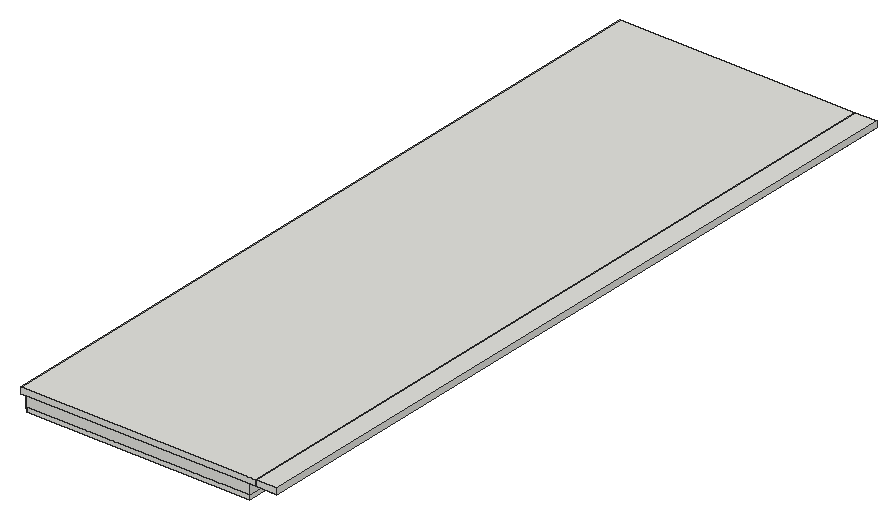
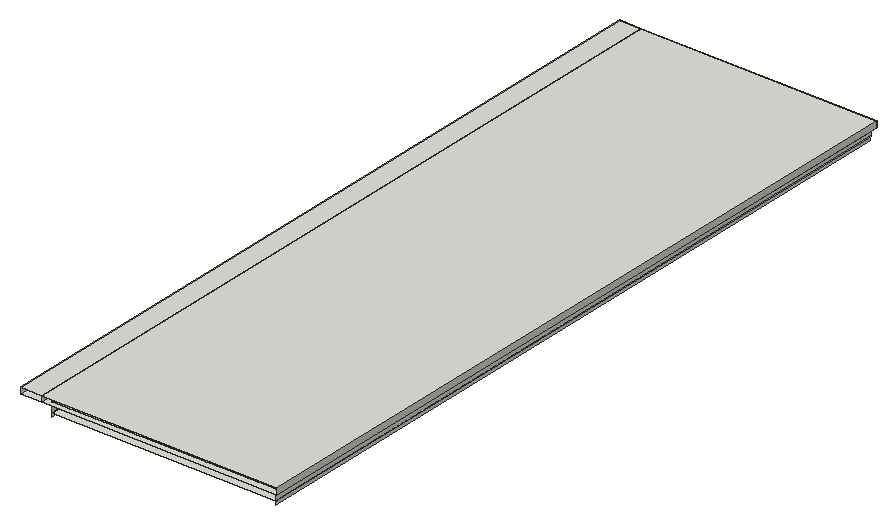
# SketchUp Ruby script. Lengths in inches.
U = 1.inch
M = Sketchup.active_model
def pt(a) = Geom::Point3d.new(a.map { |v| v * U })
def face(e, loops, mat)
  f = e.add_face(loops[0].map { |a| pt(a) })
  loops[1..].each { |l| e.add_face(l.map { |a| pt(a) }).erase! }
  f.material = f.back_material = mat if mat
  f
end
# faces: each face lists its corners as indices into pts; further lists are holes
def faces(e, pts, list, mat = nil) = list.each { |f| face(e, (f[0].is_a?(Array) ? f : [f]).map { |l| l.map { |i| pts[i] } }, mat) }
# xy, xz, yz: faces in a plane at the given z, y or x. An outline is a flat list of corners, or four numbers for a rectangle; further outlines are holes
def ring(l) = l.size == 4 ? [[l[0], l[1]], [l[2], l[1]], [l[2], l[3]], [l[0], l[3]]] : l.each_slice(2).to_a
def flat(e, list, mat, &to3) = list.each { |f| face(e, (f[0].is_a?(Array) ? f : [f]).map { |l| ring(l).map { |u, v| to3.(u, v) } }, mat) }
def xy(e, z, list, mat = nil) = flat(e, list, mat) { |x, y| [x, y, z] }
def xz(e, y, list, mat = nil) = flat(e, list, mat) { |x, z| [x, y, z] }
def yz(e, x, list, mat = nil) = flat(e, list, mat) { |y, z| [x, y, z] }
def lines(e, pts, list) = list.each { |a, b| e.add_line(pt(pts[a]), pt(pts[b])) }
# prism: a flat outline (further loops are holes) pulled along v
def prism(e, loops, v, mat = nil)
  f = face(e, loops, mat); d = Geom::Vector3d.new(v.map { |x| x * U })
  f.pushpull(f.normal.samedirection?(d) ? d.length : -d.length)
end
def box(e, o, s, mat = nil) = prism(e, [[o, [o[0] + s[0], o[1], o[2]], [o[0] + s[0], o[1] + s[1], o[2]], [o[0], o[1] + s[1], o[2]]]], [0, 0, s[2]], mat)
def at(x, y, z, deg = 0) = Geom::Transformation.translation(pt([x, y, z])) * Geom::Transformation.rotation(ORIGIN, Z_AXIS, deg.degrees)
def axes(o, x, y, z) = Geom::Transformation.new([*x, 0, *y, 0, *z, 0, *pt(o).to_a, 1])
def part(name) = M.definitions.add(name)
# library, detail: a bought-in or finely detailed component or shape, given as its bounding box
def library(name, o, s) = part(name).tap { |d| box(d.entities, o, s) }
def detail(e, o, s) = box(e.add_group.entities, o, s)
def put(e, d, t, mat = nil) = e.add_instance(d, t).tap { |i| i.material = mat if mat }
def group(e, t, mat = nil) = e.add_group.tap { |g| g.transformation = t; g.material = mat if mat }.entities
root = M.entities
xy(root,155.5,[[6,0,6.4,756.6875]])
xy(root,156.12,[[6,0,234,757.0625]])
xy(root,166.28,[[0,0,0,763.0625,240,763.0625,240,0,234,0,234,757.0625,6,757.0625,6,0],[6,0,234,757.0625],[240,0,261.625,763.0625]])
xy(root,172.28,[[0,0,240,763.0625],[240,0,261.625,763.0625]])
xz(root,0,[[6.4,152.12,234,152.12,234,156.12,6,156.12,6,155.5,6.4,155.5],[6,156.12,234,166.28],[0,166.28,240,172.28],[240,166.28,261.625,172.28]])
xz(root,551,[[57.9375,152.12,182.0625,153.65]])
yz(root,0,[[0,166.28,763.0625,172.28]])
yz(root,6,[[0,155.5,757.0625,156.12],[0,156.12,757.0625,166.28]])
yz(root,6.4,[[0,152.12,756.6875,155.5]])
yz(root,234,[[0,152.12,757.0625,156.12],[0,156.12,757.0625,166.28]])
yz(root,240,[[0,166.28,763.0625,172.28]])
yz(root,261.625,[[0,166.28,763.0625,172.28]])
p = [[59,535.0625,152.12],[57.71,535.23,152.12],[57.71,535.23,153.44],[59,535.0625,153.44],[60.29,535.23,152.12],[60.29,535.23,153.44],
  [181,535.0625,152.12],[179.71,535.23,152.12],[179.71,535.23,153.31],[181,535.0625,153.31],[182.29,535.23,152.12],[182.29,535.23,153.31],
  [56.5,535.73,152.12],[56.5,535.73,153.44],[61.5,535.73,152.12],[61.5,535.73,153.44],[178.5,535.73,152.12],[178.5,535.73,153.31],
  [183.5,535.73,152.12],[183.5,535.73,153.31],[55.46,536.53,152.12],[55.46,536.53,153.44],[62.54,536.53,152.12],[62.54,536.53,153.44],
  [177.46,536.53,152.12],[177.46,536.53,153.31],[184.54,536.53,152.12],[184.54,536.53,153.31],[54.67,537.5625,152.12],[54.67,537.5625,153.44],
  [63.33,537.5625,152.12],[63.33,537.5625,153.44],[176.67,537.5625,152.12],[176.67,537.5625,153.31],[185.33,537.5625,152.12],[185.33,537.5625,153.31],
  [54.17,538.77,152.12],[54.17,538.77,153.44],[63.83,538.77,152.12],[63.83,538.77,153.44],[176.17,538.77,152.12],[176.17,538.77,153.31],
  [185.83,538.77,152.12],[185.83,538.77,153.31],[54,540.0625,152.12],[54,540.0625,153.44],[64,540.0625,152.12],[64,540.0625,153.44],
  [176,540.0625,152.12],[176,540.0625,153.31],[186,540.0625,152.12],[186,540.0625,153.31],[54.17,541.36,152.12],[54.17,541.36,153.44],
  [63.83,541.36,152.12],[63.83,541.36,153.44],[176.17,541.36,152.12],[176.17,541.36,153.31],[185.83,541.36,152.12],[185.83,541.36,153.31],
  [54.67,542.5625,152.12],[54.67,542.5625,153.44],[63.33,542.5625,152.12],[63.33,542.5625,153.44],[176.67,542.5625,152.12],[176.67,542.5625,153.31],
  [185.33,542.5625,152.12],[185.33,542.5625,153.31],[55.46,543.6,152.12],[55.46,543.6,153.44],[62.54,543.6,152.12],[62.54,543.6,153.44],
  [177.46,543.6,152.12],[177.46,543.6,153.31],[184.54,543.6,152.12],[184.54,543.6,153.31],[56.5,544.39,152.12],[56.5,544.39,153.44],
  [61.5,544.39,152.12],[61.5,544.39,153.44],[178.5,544.39,152.12],[178.5,544.39,153.31],[183.5,544.39,152.12],[183.5,544.39,153.31],
  [57.71,544.89,152.12],[57.71,544.89,153.44],[60.29,544.89,152.12],[60.29,544.89,153.44],[179.71,544.89,152.12],[179.71,544.89,153.31],
  [182.29,544.89,152.12],[182.29,544.89,153.31],[59,545.0625,152.12],[59,545.0625,153.44],[181,545.0625,152.12],[181,545.0625,153.31],
  [54.8,551.2,152.12],[54.8,551.2,153.65],[57.9375,551,153.65],[57.9375,551,152.12],[182.0625,551,152.12],[182.0625,551,153.65],
  [185.2,551.2,153.65],[185.2,551.2,152.12],[51.72,551.82,152.12],[51.72,551.82,153.65],[188.28,551.82,153.65],[188.28,551.82,152.12],
  [48.75,552.83,152.12],[48.75,552.83,153.65],[191.25,552.83,153.65],[191.25,552.83,152.12],[45.9375,554.21,152.12],[45.9375,554.21,153.65],
  [194.0625,554.21,153.65],[194.0625,554.21,152.12],[43.33,555.96,152.12],[43.33,555.96,153.65],[196.67,555.96,153.65],[196.67,555.96,152.12],
  [40.97,558.03,152.12],[40.97,558.03,153.65],[199.03,558.03,153.65],[199.03,558.03,152.12],[38.9,560.39,152.12],[38.9,560.39,153.65],
  [201.1,560.39,153.65],[201.1,560.39,152.12],[37.15,563,152.12],[37.15,563,153.65],[202.85,563,153.65],[202.85,563,152.12],
  [35.76,565.8125,152.12],[35.76,565.8125,153.65],[204.24,565.8125,153.65],[204.24,565.8125,152.12],[34.75,568.79,152.12],[34.75,568.79,153.65],
  [205.25,568.79,153.65],[205.25,568.79,152.12],[34.14,571.87,152.12],[34.14,571.87,153.65],[205.86,571.87,153.65],[205.86,571.87,152.12],
  [23,571.0625,152.12],[21.71,571.23,152.12],[21.71,571.23,153.44],[23,571.0625,153.44],[24.29,571.23,152.12],[24.29,571.23,153.44],
  [217,571.0625,152.12],[215.71,571.23,152.12],[215.71,571.23,153.31],[217,571.0625,153.31],[218.29,571.23,152.12],[218.29,571.23,153.31],
  [20.5,571.73,152.12],[20.5,571.73,153.44],[25.5,571.73,152.12],[25.5,571.73,153.44],[214.5,571.73,152.12],[214.5,571.73,153.31],
  [219.5,571.73,152.12],[219.5,571.73,153.31],[19.46,572.53,152.12],[19.46,572.53,153.44],[26.54,572.53,152.12],[26.54,572.53,153.44],
  [213.46,572.53,152.12],[213.46,572.53,153.31],[220.54,572.53,152.12],[220.54,572.53,153.31],[33.9375,575,152.12],[33.9375,575,153.65],
  [206.0625,575,153.65],[206.0625,575,152.12],[18.67,573.5625,152.12],[18.67,573.5625,153.44],[27.33,573.5625,152.12],[27.33,573.5625,153.44],
  [212.67,573.5625,152.12],[212.67,573.5625,153.31],[221.33,573.5625,152.12],[221.33,573.5625,153.31],[18.17,574.77,152.12],[18.17,574.77,153.44],
  [27.83,574.77,152.12],[27.83,574.77,153.44],[212.17,574.77,152.12],[212.17,574.77,153.31],[221.83,574.77,152.12],[221.83,574.77,153.31],
  [18,576.0625,152.12],[18,576.0625,153.44],[28,576.0625,152.12],[28,576.0625,153.44],[212,576.0625,152.12],[212,576.0625,153.31],
  [222,576.0625,152.12],[222,576.0625,153.31],[18.17,577.36,152.12],[18.17,577.36,153.44],[27.83,577.36,152.12],[27.83,577.36,153.44],
  [212.17,577.36,152.12],[212.17,577.36,153.31],[221.83,577.36,152.12],[221.83,577.36,153.31],[18.67,578.5625,152.12],[18.67,578.5625,153.44],
  [27.33,578.5625,152.12],[27.33,578.5625,153.44],[212.67,578.5625,152.12],[212.67,578.5625,153.31],[221.33,578.5625,152.12],[221.33,578.5625,153.31],
  [19.46,579.6,152.12],[19.46,579.6,153.44],[26.54,579.6,152.12],[26.54,579.6,153.44],[213.46,579.6,152.12],[213.46,579.6,153.31],
  [220.54,579.6,152.12],[220.54,579.6,153.31],[20.5,580.39,152.12],[20.5,580.39,153.44],[25.5,580.39,152.12],[25.5,580.39,153.44],
  [214.5,580.39,152.12],[214.5,580.39,153.31],[219.5,580.39,152.12],[219.5,580.39,153.31],[21.71,580.89,152.12],[21.71,580.89,153.44],
  [24.29,580.89,152.12],[24.29,580.89,153.44],[215.71,580.89,152.12],[215.71,580.89,153.31],[218.29,580.89,152.12],[218.29,580.89,153.31],
  [23,581.0625,152.12],[23,581.0625,153.44],[185.2,551.2,155.19],[182.0625,551,155.19],[188.28,551.82,155.19],[191.25,552.83,155.19],
  [194.0625,554.21,155.19],[196.67,555.96,155.19],[199.03,558.03,155.19],[201.1,560.39,155.19],[202.85,563,155.19],[204.24,565.8125,155.19],
  [205.25,568.79,155.19],[205.86,571.87,155.19],[206.0625,575,155.19]]
faces(root,p,[[0,1,2,3],[4,0,3,5],[6,7,8,9],[10,6,9,11],[1,12,13,2],[14,4,5,15],[7,16,17,8],[18,10,11,19],
  [12,20,21,13],[22,14,15,23],[16,24,25,17],[26,18,19,27],[20,28,29,21],[30,22,23,31],[24,32,33,25],[34,26,27,35],
  [28,36,37,29],[38,30,31,39],[32,40,41,33],[42,34,35,43],[36,44,45,37],[46,38,39,47],[40,48,49,41],[50,42,43,51],
  [44,52,53,45],[54,46,47,55],[48,56,57,49],[58,50,51,59],[52,60,61,53],[62,54,55,63],[56,64,65,57],[66,58,59,67],
  [60,68,69,61],[70,62,63,71],[64,72,73,65],[74,66,67,75],[68,76,77,69],[78,70,71,79],[72,80,81,73],[82,74,75,83],
  [76,84,85,77],[86,78,79,87],[80,88,89,81],[90,82,83,91],[84,92,93,85],[92,86,87,93],[88,94,95,89],[94,90,91,95],
  [96,97,98,99],[100,101,102,103],[104,105,97,96],[103,102,106,107],[108,109,105,104],[107,106,110,111],[112,113,109,108],[111,110,114,115],
  [116,117,113,112],[115,114,118,119],[120,121,117,116],[119,118,122,123],[124,125,121,120],[123,122,126,127],[128,129,125,124],[127,126,130,131],
  [132,133,129,128],[131,130,134,135],[136,137,133,132],[135,134,138,139],[140,141,137,136],[139,138,142,143],[144,145,146,147],[148,144,147,149],
  [150,151,152,153],[154,150,153,155],[145,156,157,146],[158,148,149,159],[151,160,161,152],[162,154,155,163],[156,164,165,157],[166,158,159,167],
  [160,168,169,161],[170,162,163,171],[172,173,141,140],[143,142,174,175],[164,176,177,165],[178,166,167,179],[168,180,181,169],[182,170,171,183],
  [176,184,185,177],[186,178,179,187],[180,188,189,181],[190,182,183,191],[184,192,193,185],[194,186,187,195],[188,196,197,189],[198,190,191,199],
  [192,200,201,193],[202,194,195,203],[196,204,205,197],[206,198,199,207],[200,208,209,201],[210,202,203,211],[204,212,213,205],[214,206,207,215],
  [208,216,217,209],[218,210,211,219],[212,220,221,213],[222,214,215,223],[216,224,225,217],[226,218,219,227],[220,228,229,221],[230,222,223,231],
  [224,232,233,225],[234,226,227,235],[228,236,237,229],[238,230,231,239],[232,240,241,233],[240,234,235,241],[242,102,101,243],[244,106,102,242],
  [245,110,106,244],[246,114,110,245],[247,118,114,246],[248,122,118,247],[249,126,122,248],[250,130,126,249],[251,134,130,250],[252,138,134,251],
  [253,142,138,252],[254,174,142,253]])
